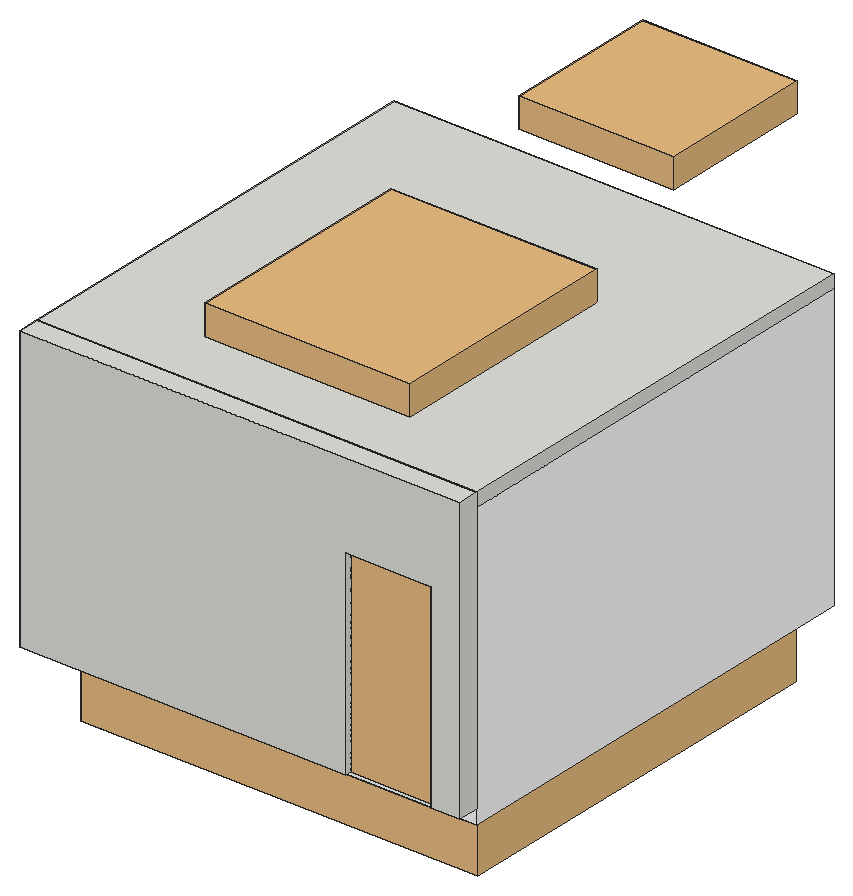
# SketchUp Ruby script. Lengths in inches.
U = 1.inch
M = Sketchup.active_model
def pt(a) = Geom::Point3d.new(a.map { |v| v * U })
def face(e, loops, mat)
  f = e.add_face(loops[0].map { |a| pt(a) })
  loops[1..].each { |l| e.add_face(l.map { |a| pt(a) }).erase! }
  f.material = f.back_material = mat if mat
  f
end
# faces: each face lists its corners as indices into pts; further lists are holes
def faces(e, pts, list, mat = nil) = list.each { |f| face(e, (f[0].is_a?(Array) ? f : [f]).map { |l| l.map { |i| pts[i] } }, mat) }
# xy, xz, yz: faces in a plane at the given z, y or x. An outline is a flat list of corners, or four numbers for a rectangle; further outlines are holes
def ring(l) = l.size == 4 ? [[l[0], l[1]], [l[2], l[1]], [l[2], l[3]], [l[0], l[3]]] : l.each_slice(2).to_a
def flat(e, list, mat, &to3) = list.each { |f| face(e, (f[0].is_a?(Array) ? f : [f]).map { |l| ring(l).map { |u, v| to3.(u, v) } }, mat) }
def xy(e, z, list, mat = nil) = flat(e, list, mat) { |x, y| [x, y, z] }
def xz(e, y, list, mat = nil) = flat(e, list, mat) { |x, z| [x, y, z] }
def yz(e, x, list, mat = nil) = flat(e, list, mat) { |y, z| [x, y, z] }
def lines(e, pts, list) = list.each { |a, b| e.add_line(pt(pts[a]), pt(pts[b])) }
# prism: a flat outline (further loops are holes) pulled along v
def prism(e, loops, v, mat = nil)
  f = face(e, loops, mat); d = Geom::Vector3d.new(v.map { |x| x * U })
  f.pushpull(f.normal.samedirection?(d) ? d.length : -d.length)
end
def box(e, o, s, mat = nil) = prism(e, [[o, [o[0] + s[0], o[1], o[2]], [o[0] + s[0], o[1] + s[1], o[2]], [o[0], o[1] + s[1], o[2]]]], [0, 0, s[2]], mat)
def at(x, y, z, deg = 0) = Geom::Transformation.translation(pt([x, y, z])) * Geom::Transformation.rotation(ORIGIN, Z_AXIS, deg.degrees)
def axes(o, x, y, z) = Geom::Transformation.new([*x, 0, *y, 0, *z, 0, *pt(o).to_a, 1])
def part(name) = M.definitions.add(name)
# library, detail: a bought-in or finely detailed component or shape, given as its bounding box
def library(name, o, s) = part(name).tap { |d| box(d.entities, o, s) }
def detail(e, o, s) = box(e.add_group.entities, o, s)
def put(e, d, t, mat = nil) = e.add_instance(d, t).tap { |i| i.material = mat if mat }
def group(e, t, mat = nil) = e.add_group.tap { |g| g.transformation = t; g.material = mat if mat }.entities
root = M.entities
M.materials.add("[0046_Gold]").color = [187, 147, 125]
M.materials.add("[Basic Tile]").color = [203, 206, 202]
M.materials.add("[Carrera Marble]").color = [207, 207, 207]
M.materials.add("[Color B08]1").color = [61, 35, 26]
M.materials.add("[Jade]").color = [111, 152, 100]
M.materials.add("[Stone Marble]").color = [143, 138, 136]
M.materials.add("indian-green-granite-stone-slab-500x500").color = [19, 53, 33]
M.materials.add("kabinet").color = [255, 255, 255]
c1 = library("Fridge\#1",[0,-2.9,0],[42,31.9,86.99])
c2 = library("HOB",[0,0,0],[20.08,29.13,2.03])
c3 = library("Geladeira Brastemp Frost Free Duplex Ative! BRM50NR - 429L -",[0,0,0],[28.11,27.02,74.41])
c4 = library("Double oven",[0,0,0],[19.88,22.8,39.15])
c5 = library("Table setting",[0,-0.06,0],[29.38,11.2,9.98])
c6 = library("dishes\#1",[-5.44,0,0],[26.06,19.72,14.48])
c7 = library("Prato decorativo",[-9.81,-1.76,0],[8.53,8.52,6.9])
c8 = library("Glass Mr Coffee Carafe",[-2.91,-2.91,-0.05],[7.03,5.82,5.83])
c9 = library("937f Haynes smg",[1.8,-9.06,2.7],[24.74,18.12,30.38])
c10 = library("AutoSave_platos BOWLS",[0,0,0],[6.24,6.24,7.68])
c11 = library("Component",[-12,-8.05,0],[20.7,16.1,16.99])
c12 = library("Kitchen Cake Stand (2)",[-6,-6,0],[12,12,6.89])
c13 = library("Pump dispenser",[0.14,17.81,0],[3.44,2.9,13.39])
c14 = library("Pump dispenser \#1",[0.14,17.81,0],[3.44,2.9,13.39])
c15 = library("Pump dispenser \#2",[0.14,17.81,0],[3.44,2.9,13.39])
c16 = library("Capped bottle",[0,0,0],[3.54,3.54,10.85])
c17 = library("Tds prts",[0,0,0],[34.14,34.14,6.01])
c18 = library("604f",[-1.28,-1.28,-3.49],[2.56,2.56,6.98])
c19 = library("model",[-1.72,-0.95,0],[3.44,1.9,7.875])
c20 = library("soya_250",[-1.1875,-1.1875,0],[2.375,2.375,7.15])
c21 = library("Sink with faucet",[0,0,0],[24.9375,22.07,25.97])
c22 = library("Olive oil bottle",[-1.12,-1.12,0],[2.24,2.24,10.75])
c23 = library("olive oil",[0,0,0],[2.33,2.33,12.9])
c24 = library("Olive bottle",[0,0,0],[2.2,2.2,10.6])
c25 = library("bowls",[-0.39,1.3,-1.14],[28.37,17.08,12.97])
c26 = part("Group308\#1")
p = [[0,0,0],[0,0,-11.43],[-4.61,0,-11.43],[30,-7,0],[-30,-7,0],[30,7,0],
  [30,0,0],[-30,7,0],[4.61,0,-11.43],[-30,0,0],[0,0,-18.5]]
lines(c26.entities,p,[[0,1],[1,2],[3,4],[5,6],[7,5],[1,8],[9,0],[0,6],[8,10],[4,9],[6,3],[2,10],
  [9,7]])
c27 = part("Rectangle Light\#6")
put(c27.entities,c26,at(0,0,0))
c28 = library("Dome Light",[-12,-12,0],[24,24,12])
c29 = library("Wooden door",[0,-2.35,-0.05],[50.61,6.5,82.92])
c30 = part("Group305\#1")
p = [[0,0,0],[0,0,-9.27],[-3.53,0,-9.27],[23,-7,0],[-23,-7,0],[23,7,0],
  [23,0,0],[-23,7,0],[3.53,0,-9.27],[-23,0,0],[0,0,-15]]
lines(c30.entities,p,[[0,1],[1,2],[3,4],[5,6],[7,5],[1,8],[9,0],[0,6],[8,10],[4,9],[6,3],[2,10],
  [9,7]])
c31 = part("Rectangle Light\#5")
put(c31.entities,c30,at(0,0,0))
c32 = part("Group\#12")
prism(c32.entities,[[[-0.02,0,0.25],[0.0625,0,0.24],[0.14,0,0.21],[0.2,0,0.15],[0.24,0,0.08],[0.25,0,0],[0.24,0,-0.08],[0.2,0,-0.15],[0.14,0,-0.21],[0.0625,0,-0.24],[-0.02,0,-0.25],[-0.1,0,-0.23],[-0.17,0,-0.18],[-0.22,0,-0.12],[-0.25,0,-0.04],[-0.25,0,0.04],[-0.22,0,0.12],[-0.17,0,0.18],[-0.1,0,0.23]]],[0,-0.125,0])
prism(c32.entities,[[[0.12,-0.125,0.15],[0.17,-0.125,0.08],[0.1875,-0.125,0],[0.17,-0.125,-0.08],[0.12,-0.125,-0.15],[0.04,-0.125,-0.18],[-0.04,-0.125,-0.18],[-0.12,-0.125,-0.15],[-0.17,-0.125,-0.08],[-0.1875,-0.125,0],[-0.17,-0.125,0.08],[-0.12,-0.125,0.15],[-0.04,-0.125,0.18],[0.04,-0.125,0.18]]],[0,-0.125,0])
c33 = library("Group\#18",[0,0,0],[27.2,23,30.82])
c34 = library("Group\#356",[0,0,0],[9.45,9.45,4.37])
c35 = library("Groupe\#1",[0,0,0],[6.09,6.09,3.67])
c36 = library("Group\#75",[0,0,0],[35.9,30.13,18.85])
c37 = library("Grupa\#8",[0,0,0],[9.45,4.72,9.45])
c38 = library("Group\#86",[0,0,0],[15.83,15.83,32.45])
c39 = library("Group\#111",[0,0,0],[51.64,51.64,108.15])
c40 = library("Group\#153",[0,0,0],[4.33,4.33,5.84])
c41 = library("Group\#154",[-3.15,-3.23,0],[20.08,20.34,20.82])
c42 = library("Group\#155",[0,0,0],[10.38,12.15,25])
c43 = library("Group\#156",[-0.21,0,0],[4.92,4.99,5.85])
c44 = library("Difference\#5",[0,12,-38.01],[168,168,66.01])
c45 = part("Difference\#2")
prism(c45.entities,[[[143,155,0],[108,155,0],[108,180,0],[168,180,0],[168,12,0],[143,12,0]],[[145.42,55.24,0],[165.27,55.24,0],[165.27,77.3125,0],[145.42,77.3125,0]]],[0,0,1])
prism(c45.entities,[[[0,180,0],[60,180,0],[60,155,0],[25,155,0],[25,42,0],[0,42,0]]],[0,0,1])
c46 = library("Group\#157",[0,0,0],[65.46,65.46,12.43])
c47 = library("Group\#17",[0,0,-1],[168,180,7])
c48 = library("Group\#27",[0,0,0.5],[86.83,98.83,24.4])
c49 = library("Group\#28",[-0.5,-0.5,0],[11.2,11.27,6])
c50 = library("Group\#29",[-0.5,-0.5,-0.1],[15,139,0.2])
c51 = library("Group\#30",[0,0,0],[60,38,52.99])
c52 = library("Group\#32",[-0.5,-0.5,0],[1,125.43,19.96])
c53 = library("Group\#33",[-0.5,-0.5,-0.1],[61,139,0.2])
xy(root,6,[[67.99,28.64,102.91,117.58]])
xy(root,6.27,[[67.99,28.64,102.91,117.58]],"[0046_Gold]")
xy(root,10,[[9,15,22,17]])
xy(root,84,[[9,15,22,17],[9,49,22,51]])
xy(root,112,[[117,188,177,189]])
xy(root,114,[[117,188,177,189]])
xz(root,15,[[9,10,22,84]],"[0046_Gold]")
xz(root,17,[[9,10,22,84]])
xz(root,28.64,[[67.99,6,102.91,6.27]])
xz(root,49,[[9,10,22,84]],"[0046_Gold]")
xz(root,51,[[9,9.96,22,69],[9,69,22,84]])
xz(root,117.58,[[67.99,6,102.91,6.27]])
xz(root,188,[[117,112,177,114]],"[0046_Gold]")
xz(root,189,[[117,112,177,114]])
yz(root,9,[[51,9.96,49,10,49,84,51,84],[15,10,17,84]])
yz(root,22,[[15,10,17,84]])
yz(root,22,[[51,9.96,51,84,49,84,49,10]],"[0046_Gold]")
yz(root,67.99,[[28.64,6,117.58,6.27]])
yz(root,102.91,[[28.64,6,117.58,6.27]])
yz(root,117,[[188,112,189,114]])
yz(root,177,[[188,112,189,114]])
p = [[9,51,9.96],[22,51,9.96],[22,49,10],[9,49,10],[9,49,84],[9,17,84],
  [9,17,10],[141.74,174.21,84.52],[141.7,174.21,84.52],[156.625,189.57,81.25],[126.7,189.57,81.25],[126.7,175,83.88]]
faces(root,p,[[0,1,2,3]])
lines(root,p,[[4,5],[6,3],[7,8],[9,10],[11,10]])
put(root,c1,axes([25.57,19.28,10],[0,0.66507,0],[-0.63,0,0],[0,0,0.81]))
put(root,c2,at(11.85,108.125,39))
put(root,c3,axes([71.55,163.5,10],[0.74131,0,0],[0,0.74025,0],[0,0,0.856]))
put(root,c4,axes([113.25,162.06,36.27],[0,1,0],[-0.89,0,0],[0,0,0.99]))
put(root,c5,at(165.86,113.53,87,-90))
put(root,c6,at(153.68,165.39,39))
put(root,c7,axes([123.27,175.01,103.75],[0.12678,-1.13031,0],[1.13031,0.12678,0],[0,0,1.1374]))
put(root,c8,at(146.5625,180.08,92.5))
put(root,c9,axes([151.7,179.53,91.72],[0.28012,-0.07506,0],[0.07506,0.28012,0],[0,0,0.29]))
put(root,c10,at(120.62,174.12,81.25),"[Jade]")
put(root,c10,at(127.29,175,81.25),"[Jade]")
put(root,c11,axes([125.3,186.47,70],[0.24,0,0],[0,0.24,0],[0,0,0.24]))
put(root,c11,axes([130.6,186.47,70],[0.24,0,0],[0,0.24,0],[0,0,0.24]))
put(root,c11,axes([125.41,181.88,70],[0.24,0,0],[0,0.24,0],[0,0,0.24]))
put(root,c11,axes([130.7,181.88,70],[0.24,0,0],[0,0.24,0],[0,0,0.24]))
put(root,c11,axes([126.15,176.93,70],[0.24,0,0],[0,0.24,0],[0,0,0.24]))
put(root,c11,axes([131.45,176.93,70],[0.24,0,0],[0,0.24,0],[0,0,0.24]))
put(root,c12,at(125.24,181.75,92.5))
put(root,c13,at(191.09,112.2,68.75,90))
put(root,c14,at(194.87,112.2,68.75,90))
put(root,c15,at(187.57,112.2,68.75,90))
put(root,c16,at(142.99,168.55,39))
put(root,c16,at(143.92,175.48,39))
put(root,c17,axes([135.7,179.34,82.64],[0.264,0,0],[0,0.264,0],[0,0,0.264]),"indian-green-granite-stone-slab-500x500")
put(root,c17,axes([135.7,179.32,81.25],[0.264,0,0],[0,0.264,0],[0,0,0.264]))
put(root,c17,axes([135.72,179.24,83.78],[0.264,0,0],[0,0.264,0],[0,0,0.264]),"indian-green-granite-stone-slab-500x500")
put(root,c18,at(167.125,38.66,43.8125))
put(root,c19,at(170.95,37.99,39))
put(root,c20,at(168.15,44.38,39))
put(root,c6,axes([163,86.36,69],[0,-0.53,0],[0.53,0,0],[0,0,0.53]),"[0046_Gold]")
put(root,c21,axes([174.39,64.18,30.29],[0,0.89,0],[-0.89,0,0],[0,0,0.89]))
put(root,c22,at(13.93,177.46,39))
put(root,c23,at(17.39,178.54,39))
put(root,c24,at(10.24,173.49,39))
put(root,c25,at(11.8,87.1,40.14,-90))
put(root,c27,axes([147,186.5,101.7],[1,0,0],[0,0.3567,0],[0,0,0.18]))
put(root,c27,axes([147,186.5,90.46],[1,0,0],[0,0.3567,0],[0,0,0.18]))
put(root,c27,axes([147,186.5,79.21],[1,0,0],[0,0.3567,0],[0,0,0.18]))
put(root,c27,axes([147,186.5,68.96],[1,0,0],[0,0.3567,0],[0,0,0.18]))
put(root,c28,at(123.78,182.05,111))
put(root,c29,axes([138,4.6875,6],[0.71131,0,0],[0,1,0],[0,0,1.01361]))
g1 = group(root,at(9,9,0),"kabinet")
xy(g1,0,[[0,0,168,180]])
xy(g1,6,[[0,0,168,180]],"[Basic Tile]")
xz(g1,0,[[0,0,168,6]])
xz(g1,180,[[0,0,168,6]])
yz(g1,0,[[0,0,180,6]])
yz(g1,168,[[0,0,180,6]])
g2 = group(root,at(9,9,6),"[0046_Gold]")
prism(g2,[[[148,160,0],[20,160,0],[20,41.74,0],[16.25,41.74,0],[16.25,6,0],[0,6,0],[0,180,0],[168,180,0],[168,12,0],[148,12,0]]],[0,0,4])
g3 = group(root,at(0,9,0),"kabinet")
xy(g3,0,[[0,0,0,189,186,189,186,0,177,0,177,180,9,180,9,0]])
xy(g3,120,[[0,0,9,0,9,180,177,180,177,0,186,0,186,189,0,189]])
xz(g3,0,[[0,0,9,120],[177,0,186,120]])
xz(g3,180,[[9,0,177,120]],"[Carrera Marble]")
xz(g3,189,[[0,0,186,120]])
yz(g3,0,[[0,0,189,120]])
yz(g3,9,[[0,0,180,120]],"[Carrera Marble]")
yz(g3,177,[[0,0,180,120]])
yz(g3,186,[[0,0,189,120]])
g4 = group(root,at(9,15,96),"[0046_Gold]")
xy(g4,0,[[0,0,0,174,14,174,14,151.62,13,151.62,13,151.38,14,151.38,14,126.12,13,126.12,13,125.88,14,125.88,14,90.12,13,90.12,13,89.88,14,89.88,14,72.12,13,72.12,13,71.88,14,71.88,14,36.12,13,36.12,13,35.88,14,35.88,14,18.06,13,18.06,13,17.82,14,17.82,14,0]])
xy(g4,18,[[0,0,14,0,14,17.82,13,17.82,13,18.06,14,18.06,14,35.88,13,35.88,13,36.12,14,36.12,14,71.88,13,71.88,13,72.12,14,72.12,14,89.88,13,89.88,13,90.12,14,90.12,14,125.88,13,125.88,13,126.12,14,126.12,14,151.38,13,151.38,13,151.62,14,151.62,14,174,0,174]])
xz(g4,0,[[0,0,14,18]])
xz(g4,17.82,[[13,0,14,18]])
xz(g4,18.06,[[13,0,14,18]])
xz(g4,35.88,[[13,0,14,18]])
xz(g4,36.12,[[13,0,14,18]])
xz(g4,71.88,[[13,0,14,18]])
xz(g4,72.12,[[13,0,14,18]])
xz(g4,89.88,[[13,0,14,18]])
xz(g4,90.12,[[13,0,14,18]])
xz(g4,125.88,[[13,0,14,18]])
xz(g4,126.12,[[13,0,14,18]])
xz(g4,151.38,[[13,0,14,18]])
xz(g4,151.62,[[13,0,14,18]])
xz(g4,174,[[0,0,14,18]])
yz(g4,0,[[0,0,36,18],[126,0,174,18]])
yz(g4,13,[[17.82,0,18.06,18],[35.88,0,36.12,18],[71.88,0,72.12,18],[89.88,0,90.12,18],[125.88,0,126.12,18],
  [151.38,0,151.62,18]])
yz(g4,14,[[0,0,17.82,18],[18.06,0,35.88,18],[36.12,0,71.88,18],[72.12,0,89.88,18],[90.12,0,125.88,18],
  [126.12,0,151.38,18],[151.62,0,174,18]])
g5 = group(root,at(9,51,69))
xy(g5,0,[[0,0,0,53.88,14,53.88,14,36.12,13,36.12,13,35.88,14,35.88,14,18.12,13,18.12,13,17.88,14,17.88,14,0],[0,90.12,0,138,14,138,14,123.12,13,123.12,13,122.88,14,122.88,14,108.12,13,108.12,13,107.88,14,107.88,14,90.12]])
xy(g5,16.625,[[0,53.88,0,90.12,13,90.12,13,89.88,14,89.88,14,54.12,13,54.12,13,53.88]])
xy(g5,27,[[0,0,14,0,14,17.88,13,17.88,13,18.12,14,18.12,14,35.88,13,35.88,13,36,0,36],[0,36,13,36,13,36.12,14,36.12,14,53.88,13,53.88,13,54,0,54],[0,54,13,54,13,54.12,14,54.12,14,89.88,13,89.88,13,90,0,90],[0,90,13,90,13,90.12,14,90.12,14,107.88,13,107.88,13,108.12,14,108.12,14,122.88,13,122.88,13,123.12,14,123.12,14,138,0,138]])
xz(g5,0,[[0,0,14,27]])
xz(g5,17.88,[[13,0,14,27]])
xz(g5,18.12,[[13,0,14,27]])
xz(g5,35.88,[[13,0,14,27]])
xz(g5,36.12,[[13,0,14,27]])
xz(g5,53.88,[[0,0,13,16.625],[13,0,14,27]])
xz(g5,54.12,[[13,16.625,14,27]])
xz(g5,89.88,[[13,16.625,14,27]])
xz(g5,90.12,[[0,0,13,16.625],[13,0,14,27]])
xz(g5,107.88,[[13,0,14,27]])
xz(g5,108.12,[[13,0,14,27]])
xz(g5,122.88,[[13,0,14,27]])
xz(g5,123.12,[[13,0,14,27]])
xz(g5,138,[[0,0,14,27]])
yz(g5,0,[[0,0,36,27],[36,0,36,27,54,27,54,16.625,53.88,16.625,53.88,0],[90,0,90.12,16.625],[54,16.625,90,27]])
yz(g5,13,[[17.88,0,18.12,27],[35.88,0,36.12,27],[107.88,0,108.12,27],[122.88,0,123.12,27],[53.88,16.625,54.12,27],
  [89.88,16.625,90.12,27]])
yz(g5,14,[[0,0,17.88,27],[18.12,0,35.88,27],[36.12,0,53.88,27],[90.12,0,107.88,27],[108.12,0,122.88,27],
  [123.12,0,138,27],[54.12,16.625,89.88,27]])
g6 = group(root,at(9,15,84),"[0046_Gold]")
xy(g6,0,[[0,0,14,36]])
xy(g6,2,[[13,0.76,14,36]])
xy(g6,12,[[0,0,14,0,14,0.76,13,0.76,13,36,0,36]])
xz(g6,0,[[0,0,14,12]])
xz(g6,0.76,[[13,2,14,12]])
xz(g6,36,[[0,0,0,12,13,12,13,2,14,2,14,0]])
yz(g6,0,[[0,0,36,12]])
yz(g6,13,[[0.76,2,36,12]])
yz(g6,14,[[0,0,36,0,36,2,0.76,2,0.76,12,0,12]])
g7 = group(root,at(23,175,69),"kabinet")
xy(g7,0,[[0,0,0,14,46,14,46,0,23.12,0,23.12,1,22.88,1,22.88,0]])
xy(g7,26.88,[[0,0,22.88,1],[23.12,0,46,1]])
xy(g7,27.12,[[0,0,22.88,1],[23.12,0,46,1]])
xy(g7,45,[[0,0,22.88,0,22.88,1,23.12,1,23.12,0,46,0,46,14,0,14]])
xz(g7,0,[[0,0,22.88,26.88],[23.12,0,46,26.88]])
xz(g7,0,[[0,27.12,22.88,45],[23.12,27.12,46,45]],"[0046_Gold]")
xz(g7,1,[[22.88,0,23.12,26.88],[0,26.88,46,27.12],[22.88,27.12,23.12,45]])
xz(g7,14,[[0,27,46,45]])
yz(g7,0,[[0,0,0,26.88,1,26.88,1,27,14,27,14,0],[1,27,1,27.12,0,27.12,0,45,14,45,14,27]])
yz(g7,22.88,[[0,0,1,26.88],[0,27.12,1,45]])
yz(g7,23.12,[[0,0,1,26.88],[0,27.12,1,45]])
yz(g7,46,[[0,0,14,0,14,27,1,27,1,26.88,0,26.88],[1,27,14,27,14,45,0,45,0,27.12,1,27.12]])
put(g7,c31,axes([23,3.5,-0.05],[1,0,0],[0,0.5,0],[0,0,0.72]))
g8 = group(root,at(69,159,10),"[0046_Gold]")
xy(g8,0,[[0,0,2,30],[46,0,48,30]])
xy(g8,70,[[2,0,46,30]])
xy(g8,71,[[2,0,46,0,46,1,24.12,1,24.12,2,23.88,2,23.88,1,2,1]])
xy(g8,102,[[2,0,23.88,1],[23.88,0,24.12,2],[24.12,0,46,1]])
xy(g8,104,[[0,0,48,30]])
xz(g8,0,[[[0,0,2,0,2,70,46,70,46,0,48,0,48,104,0,104],[2,71,46,102]]])
xz(g8,1,[[2,71,23.88,102],[24.12,71,46,102]])
xz(g8,2,[[23.88,71,24.12,102]])
xz(g8,30,[[0,0,0,104,48,104,48,0,46,0,46,70,2,70,2,0]])
yz(g8,0,[[0,0,30,104]])
yz(g8,2,[[0,0,30,70],[0,71,1,102]])
yz(g8,23.88,[[1,71,2,102]])
yz(g8,24.12,[[1,71,2,102]])
yz(g8,46,[[0,0,30,70],[0,71,1,102]])
yz(g8,48,[[0,0,30,104]])
g9 = group(root,at(93.13,159,10),"[0046_Gold]")
box(g9,[0,0,0],[21.87,30,26.27])
g10 = group(root,at(7.2,111.6,78.04))
xz(g10,0,[[[0.331,0.021,0.38,0.024,0.427,0.036,0.472,0.055,0.514,0.08,0.551,0.112,0.582,0.149,0.608,0.191,0.626,0.237,0.638,0.284,0.642,0.333,0.638,0.382,0.626,0.43,0.608,0.475,0.582,0.517,0.551,0.554,0.514,0.586,0.472,0.612,0.427,0.631,0.38,0.642,0.331,0.646,0.282,0.642,0.19,0.612,0.157,0.592,0.148,0.586,0.13,0.57,0.111,0.554,0.08,0.517,0.054,0.475,0.036,0.43,0.024,0.382,0.02,0.333,0.024,0.284,0.036,0.237,0.054,0.191,0.08,0.149,0.111,0.112,0.148,0.08,0.19,0.055,0.235,0.036,0.282,0.024],[0.331,0.037,0.285,0.041,0.24,0.052,0.198,0.069,0.25,0.053,0.289,0.047,0.317,0.047,0.34,0.049,0.356,0.058,0.366,0.067,0.37,0.076,0.37,0.085,0.366,0.096,0.356,0.104,0.341,0.104,0.334,0.099,0.317,0.086,0.29,0.076,0.245,0.076,0.194,0.09,0.144,0.115,0.118,0.137,0.077,0.18,0.051,0.242,0.041,0.287,0.037,0.333,0.041,0.38,0.051,0.427,0.057,0.4375,0.055,0.419,0.049,0.398,0.047,0.345,0.05,0.324,0.06,0.306,0.069,0.298,0.081,0.293,0.093,0.296,0.103,0.306,0.103,0.325,0.088,0.342,0.075,0.373,0.075,0.419,0.079,0.436,0.094,0.481,0.113,0.516,0.138,0.55,0.186,0.593,0.24,0.615,0.285,0.626,0.331,0.629,0.377,0.626,0.424,0.615,0.465,0.597,0.504,0.573,0.424,0.61,0.417,0.61,0.399,0.615,0.38,0.618,0.335,0.618,0.32,0.615,0.303,0.604,0.294,0.594,0.294,0.583,0.297,0.569,0.306,0.562,0.321,0.562,0.346,0.58,0.367,0.589,0.384,0.591,0.404,0.591,0.426,0.587,0.451,0.581,0.501,0.561,0.544,0.529,0.574,0.496,0.593,0.469,0.611,0.425,0.622,0.38,0.625,0.333,0.622,0.287,0.611,0.242,0.593,0.199,0.612,0.26,0.616,0.276,0.616,0.328,0.606,0.358,0.589,0.37,0.571,0.37,0.56,0.357,0.56,0.346,0.563,0.335,0.572,0.327,0.581,0.311,0.584,0.299,0.589,0.288,0.589,0.252,0.566,0.178,0.55,0.148,0.532,0.124,0.513,0.103,0.495,0.088,0.465,0.069,0.422,0.052,0.377,0.041]],[[0.331,0.037,0.377,0.041,0.422,0.052,0.465,0.069,0.495,0.088,0.513,0.103,0.532,0.124,0.55,0.148,0.566,0.178,0.589,0.252,0.589,0.288,0.584,0.299,0.581,0.311,0.572,0.327,0.563,0.335,0.56,0.346,0.56,0.357,0.571,0.37,0.589,0.37,0.606,0.358,0.616,0.328,0.616,0.276,0.612,0.26,0.593,0.199,0.611,0.242,0.622,0.287,0.625,0.333,0.622,0.38,0.611,0.425,0.593,0.469,0.574,0.496,0.544,0.529,0.501,0.561,0.451,0.581,0.426,0.587,0.404,0.591,0.384,0.591,0.367,0.589,0.346,0.58,0.321,0.562,0.306,0.562,0.297,0.569,0.294,0.583,0.294,0.594,0.303,0.604,0.32,0.615,0.335,0.618,0.38,0.618,0.399,0.615,0.417,0.61,0.424,0.61,0.504,0.573,0.465,0.597,0.424,0.615,0.377,0.626,0.331,0.629,0.285,0.626,0.24,0.615,0.186,0.593,0.138,0.55,0.113,0.516,0.094,0.481,0.079,0.436,0.075,0.419,0.075,0.373,0.088,0.342,0.103,0.325,0.103,0.306,0.093,0.296,0.081,0.293,0.069,0.298,0.06,0.306,0.05,0.324,0.047,0.345,0.049,0.398,0.055,0.419,0.057,0.4375,0.051,0.427,0.041,0.38,0.037,0.333,0.041,0.287,0.051,0.242,0.077,0.18,0.118,0.137,0.144,0.115,0.194,0.09,0.245,0.076,0.29,0.076,0.317,0.086,0.334,0.099,0.341,0.104,0.356,0.104,0.366,0.096,0.37,0.085,0.37,0.076,0.366,0.067,0.356,0.058,0.34,0.049,0.317,0.047,0.289,0.047,0.25,0.053,0.198,0.069,0.24,0.052,0.285,0.041],[0.22,0.163,0.187,0.164,0.166,0.177,0.156,0.194,0.153,0.215,0.159,0.241,0.173,0.265,0.189,0.283,0.26,0.327,0.28,0.336,0.283,0.343,0.283,0.354,0.28,0.354,0.258,0.343,0.247,0.343,0.228,0.347,0.215,0.362,0.208,0.377,0.192,0.381,0.177,0.396,0.17,0.413,0.17,0.441,0.177,0.461,0.185,0.465,0.192,0.46,0.187,0.448,0.189,0.42,0.191,0.414,0.203,0.401,0.208,0.401,0.208,0.414,0.21,0.427,0.225,0.463,0.241,0.487,0.264,0.505,0.276,0.508,0.294,0.508,0.308,0.496,0.312,0.486,0.312,0.47,0.307,0.453,0.29,0.423,0.277,0.41,0.265,0.397,0.249,0.386,0.236,0.381,0.236,0.373,0.249,0.364,0.255,0.364,0.267,0.368,0.286,0.38,0.298,0.409,0.307,0.424,0.318,0.432,0.331,0.432,0.334,0.426,0.332,0.41,0.31,0.382,0.308,0.377,0.305,0.353,0.311,0.353,0.337,0.37,0.351,0.378,0.364,0.387,0.378,0.398,0.378,0.441,0.388,0.466,0.4,0.487,0.429,0.508,0.452,0.508,0.466,0.498,0.472,0.483,0.472,0.468,0.465,0.449,0.451,0.43,0.435,0.414,0.41,0.394,0.41,0.386,0.42,0.375,0.463,0.375,0.47,0.37,0.47,0.362,0.464,0.353,0.457,0.351,0.417,0.351,0.396,0.339,0.379,0.322,0.372,0.303,0.364,0.272,0.364,0.252,0.373,0.223,0.389,0.202,0.414,0.189,0.445,0.189,0.475,0.213,0.479,0.221,0.483,0.238,0.483,0.255,0.482,0.262,0.474,0.279,0.464,0.288,0.45,0.292,0.434,0.285,0.428,0.275,0.428,0.262,0.438,0.243,0.441,0.233,0.437,0.227,0.423,0.227,0.411,0.236,0.402,0.252,0.401,0.28,0.417,0.303,0.431,0.311,0.454,0.316,0.476,0.31,0.493,0.296,0.502,0.282,0.51,0.262,0.51,0.227,0.503,0.212,0.494,0.191,0.477,0.177,0.458,0.166,0.446,0.163,0.408,0.163,0.387,0.171,0.371,0.181,0.351,0.201,0.338,0.234,0.334,0.26,0.334,0.272,0.339,0.296,0.347,0.317,0.36,0.335,0.385,0.358,0.399,0.365,0.39,0.378,0.33,0.34,0.304,0.325,0.304,0.308,0.297,0.257,0.284,0.218,0.267,0.192,0.244,0.172]],[[0.22,0.163,0.244,0.172,0.267,0.192,0.284,0.218,0.297,0.257,0.304,0.308,0.304,0.325,0.33,0.34,0.39,0.378,0.399,0.365,0.385,0.358,0.36,0.335,0.347,0.317,0.339,0.296,0.334,0.272,0.334,0.26,0.338,0.234,0.351,0.201,0.371,0.181,0.387,0.171,0.408,0.163,0.446,0.163,0.458,0.166,0.477,0.177,0.494,0.191,0.503,0.212,0.51,0.227,0.51,0.262,0.502,0.282,0.493,0.296,0.476,0.31,0.454,0.316,0.431,0.311,0.417,0.303,0.401,0.28,0.402,0.252,0.411,0.236,0.423,0.227,0.437,0.227,0.441,0.233,0.438,0.243,0.428,0.262,0.428,0.275,0.434,0.285,0.45,0.292,0.464,0.288,0.474,0.279,0.482,0.262,0.483,0.255,0.483,0.238,0.479,0.221,0.475,0.213,0.445,0.189,0.414,0.189,0.389,0.202,0.373,0.223,0.364,0.252,0.364,0.272,0.372,0.303,0.379,0.322,0.396,0.339,0.417,0.351,0.457,0.351,0.464,0.353,0.47,0.362,0.47,0.37,0.463,0.375,0.42,0.375,0.41,0.386,0.41,0.394,0.435,0.414,0.451,0.43,0.465,0.449,0.472,0.468,0.472,0.483,0.466,0.498,0.452,0.508,0.429,0.508,0.4,0.487,0.388,0.466,0.378,0.441,0.378,0.398,0.364,0.387,0.351,0.378,0.337,0.37,0.311,0.353,0.305,0.353,0.308,0.377,0.31,0.382,0.332,0.41,0.334,0.426,0.331,0.432,0.318,0.432,0.307,0.424,0.298,0.409,0.286,0.38,0.267,0.368,0.255,0.364,0.249,0.364,0.236,0.373,0.236,0.381,0.249,0.386,0.265,0.397,0.277,0.41,0.29,0.423,0.307,0.453,0.312,0.47,0.312,0.486,0.308,0.496,0.294,0.508,0.276,0.508,0.264,0.505,0.241,0.487,0.225,0.463,0.21,0.427,0.208,0.414,0.208,0.401,0.203,0.401,0.191,0.414,0.189,0.42,0.187,0.448,0.192,0.46,0.185,0.465,0.177,0.461,0.17,0.441,0.17,0.413,0.177,0.396,0.192,0.381,0.208,0.377,0.215,0.362,0.228,0.347,0.247,0.343,0.258,0.343,0.28,0.354,0.283,0.354,0.283,0.343,0.28,0.336,0.26,0.327,0.189,0.283,0.173,0.265,0.159,0.241,0.153,0.215,0.156,0.194,0.166,0.177,0.187,0.164],[0.198,0.191,0.188,0.198,0.184,0.206,0.185,0.222,0.189,0.238,0.2,0.252,0.207,0.264,0.243,0.292,0.271,0.31,0.278,0.312,0.27,0.274,0.26,0.241,0.245,0.215,0.22,0.191],[0.235,0.406,0.235,0.427,0.244,0.45,0.259,0.474,0.271,0.483,0.282,0.486,0.287,0.481,0.287,0.47,0.281,0.455,0.268,0.433,0.249,0.414],[0.407,0.42,0.403,0.423,0.405,0.431,0.405,0.441,0.409,0.453,0.418,0.472,0.43,0.483,0.441,0.486,0.447,0.481,0.447,0.469,0.436,0.447,0.425,0.436,0.414,0.424]],[0.198,0.191,0.22,0.191,0.245,0.215,0.26,0.241,0.27,0.274,0.278,0.312,0.271,0.31,0.243,0.292,0.207,0.264,0.2,0.252,0.189,0.238,0.185,0.222,0.184,0.206,0.188,0.198],[0.235,0.406,0.249,0.414,0.268,0.433,0.281,0.455,0.287,0.47,0.287,0.481,0.282,0.486,0.271,0.483,0.259,0.474,0.244,0.45,0.235,0.427],
  [0.407,0.42,0.414,0.424,0.425,0.436,0.436,0.447,0.447,0.469,0.447,0.481,0.441,0.486,0.43,0.483,0.418,0.472,0.409,0.453,0.405,0.441,0.405,0.431,0.403,0.423]])
xz(g10,0.016,[[0.331,0,0.417,0.011,0.497,0.045,0.565,0.098,0.618,0.167,0.651,0.247,0.662,0.333,0.651,0.42,0.618,0.5,0.565,0.569,0.497,0.622,0.417,0.655,0.331,0.667,0.245,0.655,0.166,0.622,0.097,0.569,0.044,0.5,0.011,0.42,0,0.333,0.011,0.247,0.044,0.167,0.097,0.098,0.166,0.045,0.245,0.011],[1.415,0.03,1.465,0.03,1.465,0.038,1.478,0.038,1.51,0.08,1.542,0.19,1.571,0.318,1.573,0.334,1.681,0.332,1.681,0.36,1.585,0.36,1.589,0.389,1.604,0.443,1.625,0.468,1.649,0.468,1.665,0.443,1.687,0.443,1.693,0.448,1.693,0.464,1.682,0.487,1.662,0.49,1.662,0.495,1.632,0.495,1.592,0.478,1.56,0.446,1.542,0.396,1.532,0.36,1.487,0.36,1.487,0.332,1.527,0.332,1.506,0.244,1.486,0.171,1.47,0.09,1.453,0.048,1.431,0.065,1.431,0.076,1.397,0.076,1.397,0.047],[1.733,0.146,1.756,0.193,1.819,0.456,1.819,0.475,1.829,0.475,1.829,0.489,1.782,0.488,1.782,0.483,1.738,0.483,1.738,0.461,1.77,0.461,1.77,0.432,1.708,0.198,1.708,0.176],[1.733,0.146,1.763,0.147,1.808,0.192,1.808,0.212,1.815,0.212,1.815,0.232,1.795,0.232,1.795,0.216,1.763,0.173,1.759,0.173,1.751,0.182],[[0.853,0.147,0.995,0.147,0.995,0.168,0.976,0.168,0.976,0.174,0.963,0.174,0.963,0.21,0.99,0.3,1.077,0.3,1.127,0.314,1.153,0.341,1.168,0.362,1.168,0.421,1.115,0.463,1.032,0.471,0.933,0.471,0.933,0.45,0.964,0.443,0.964,0.411,0.893,0.173,0.872,0.173,0.872,0.167,0.861,0.167,0.861,0.16,0.853,0.16],[0.995,0.316,1.033,0.446,1.084,0.442,1.11,0.408,1.11,0.383,1.1,0.358,1.074,0.331,1.041,0.316]],
  [1.154,0.147,1.204,0.147,1.248,0.286,1.278,0.329,1.289,0.329,1.295,0.314,1.305,0.315,1.305,0.308,1.316,0.308,1.316,0.314,1.335,0.324,1.335,0.348,1.327,0.348,1.327,0.36,1.309,0.36,1.309,0.368,1.295,0.368,1.295,0.361,1.28,0.361,1.252,0.337,1.252,0.327,1.238,0.315,1.238,0.345,1.219,0.365,1.196,0.365,1.196,0.36,1.182,0.36,1.163,0.34,1.143,0.304,1.143,0.294,1.133,0.294,1.133,0.281,1.158,0.281,1.184,0.334,1.194,0.334,1.194,0.272],[[1.344,0.148,1.409,0.148,1.441,0.164,1.457,0.186,1.472,0.21,1.486,0.245,1.486,0.321,1.457,0.353,1.457,0.36,1.442,0.36,1.442,0.367,1.394,0.367,1.394,0.359,1.38,0.359,1.352,0.338,1.326,0.306,1.31,0.272,1.31,0.25,1.302,0.25,1.302,0.191,1.319,0.168],[1.361,0.168,1.349,0.196,1.349,0.217,1.355,0.217,1.355,0.248,1.377,0.304,1.394,0.333,1.406,0.349,1.419,0.349,1.444,0.332,1.444,0.279,1.429,0.231,1.412,0.19,1.39,0.168]],[[1.863,0.148,1.914,0.148,1.949,0.169,1.968,0.191,1.974,0.198,1.982,0.208,1.982,0.222,1.968,0.222,1.968,0.234,1.959,0.228,1.959,0.214,1.926,0.18,1.908,0.172,1.886,0.172,1.88,0.183,1.878,0.23,1.925,0.244,1.962,0.268,2,0.31,2,0.341,1.976,0.366,1.929,0.366,1.891,0.34,1.861,0.308,1.836,0.264,1.836,0.238,1.826,0.238,1.826,0.191],[1.899,0.262,1.891,0.264,1.908,0.307,1.932,0.34,1.943,0.347,1.956,0.347,1.965,0.317,1.948,0.3,1.922,0.27,1.915,0.265,1.912,0.262]],[1.611,0.153,1.655,0.153,1.68,0.176,1.701,0.216,1.701,0.239,1.685,0.239,1.675,0.209,1.675,0.2,1.649,0.179,1.649,0.228,1.681,0.332,1.627,0.333,1.597,0.212,1.597,0.174],[1.661,0.371,1.674,0.371,1.692,0.391,1.692,0.406,1.68,0.425,1.656,0.425,1.643,0.41,1.643,0.387]])
g11 = group(root,at(12.9375,134.81,77.72))
xy(g11,0,[[0,-4.78,0.71,-2.39],[0.71,-4.78,1.42,-2.39],[0,-2.39,1.42,0]])
p = [[0,-4.78,0],[0,-4.78,2.25]]
lines(g11,p,[[0,1]])
g12 = group(root,at(12.92,129.48,77.8))
put(g12,c32,axes([-2,-17.76,0.75],[1.00684,0,0],[0,1,0],[0,0,1.00344]))
put(g12,c32,axes([2,-17.76,0.75],[1.00684,0,0],[0,1,0],[0,0,1.00344]))
put(g12,c32,axes([-1,-17.76,0.75],[1.00684,0,0],[0,1,0],[0,0,1.00344]))
put(g12,c32,axes([0,-17.76,0.75],[1.00684,0,0],[0,1,0],[0,0,1.00344]))
put(g12,c32,axes([1,-17.76,0.75],[1.00684,0,0],[0,1,0],[0,0,1.00344]))
put(root,c33,at(1.91,108.86,81.92),"[0046_Gold]")
put(root,c34,axes([131.65,176.64,103.75],[1,0,0],[0,1,0],[0,0,1.41]),"[Color B08]1")
put(root,c35,axes([132.4375,180.34,92.5],[1.16047,-0.67,0],[0.67,1.16047,0],[0,0,1.8492]))
put(root,c36,axes([143.68,175,70],[0.44,0,0],[0,0.44,0],[0,0,0.3847]))
put(root,c37,at(169.84,61.01,87,-90))
put(root,c38,axes([56.5,181.95,39],[0.18154,0,0],[0,0.18154,0],[0,0,0.18444]))
put(root,c38,axes([56.31,175.83,39],[0.18154,0,0],[0,0.18154,0],[0,0,0.18444]))
put(root,c38,axes([56.32,171.49,39],[0.18154,0,0],[0,0.18154,0],[0,0,0.18444]))
put(root,c38,axes([59.79,175.88,39],[0.18154,0,0],[0,0.18154,0],[0,0,0.18444]))
put(root,c38,axes([59.8,171.54,39],[0.18154,0,0],[0,0.18154,0],[0,0,0.18444]))
put(root,c38,axes([59.98,182,39],[0.18154,0,0],[0,0.18154,0],[0,0,0.18444]))
put(root,c38,axes([62.99,176.18,39],[0.18154,0,0],[0,0.18154,0],[0,0,0.18444]))
put(root,c38,axes([63,171.84,39],[0.18154,0,0],[0,0.18154,0],[0,0,0.18444]))
put(root,c38,axes([63.18,182.3,39],[0.18154,0,0],[0,0.18154,0],[0,0,0.18444]))
put(root,c39,axes([170.01,66.32,87],[0,-0.09987,0],[0.09987,0,0],[0,0,0.09975]))
put(root,c39,axes([126.41,181.64,39],[0.09987,0,0],[0,0.09987,0],[0,0,0.09975]))
put(root,c37,at(131.72,181.47,39))
put(root,c34,axes([166.19,58,68.39],[1,0,0],[0,1,0],[0,0,1.41]),"[Color B08]1")
put(root,c40,at(169.76,71.62,87))
put(root,c41,axes([158.46,130.1875,39],[0.75,0,0],[0,0.75,0],[0,0,0.75]))
put(root,c42,axes([164.7,121.06,39],[0.73,0,0],[0,0.73,0],[0,0,0.73]))
put(root,c43,at(165.73,99.05,69))
put(root,c44,at(9,9,10),"[0046_Gold]")
put(root,c45,at(9,9,38),"[Stone Marble]")
put(root,c46,at(97.65,141.85,174.375))
g13 = group(root,at(0,9,120))
box(g13,[0,0,0],[186,189,6])
put(root,c47,axes([23,9,114.0625],[0.83283,0,0],[0,0.83889,0],[0,0,1]))
put(root,c48,at(50.09,35.03,113.5625))
put(root,c49,at(87.86,144.71,114.0625))
put(root,c50,at(9,51,69))
put(root,c51,at(117,151,61.01))
g14 = group(root,at(163,21,67))
xy(g14,0,[[0,0,14,124.43]],"[0046_Gold]")
xy(g14,2,[[0,0,14,124.43]],"[0046_Gold]")
xy(g14,18,[[0,0,14,124.43]],"[0046_Gold]")
xy(g14,20,[[0,0,14,124.43]],"[0046_Gold]")
xz(g14,0,[[0,0,14,2],[0,18,14,20]],"[0046_Gold]")
xz(g14,124.43,[[0,0,14,2],[0,18,14,20]])
yz(g14,0,[[0,0,124.43,2],[0,18,124.43,20]],"[0046_Gold]")
yz(g14,14,[[0,0,124.43,2],[0,18,124.43,20]])
put(root,c52,at(177,21,65))
put(root,c53,at(9,51,9.96))
g15 = group(root,at(0,0,6))
prism(g15,[[[0,0,0],[138,0,0],[138,0,84],[174,0,84],[174,0,0],[186,0,0],[186,0,120],[0,0,120]]],[0,9,0])
